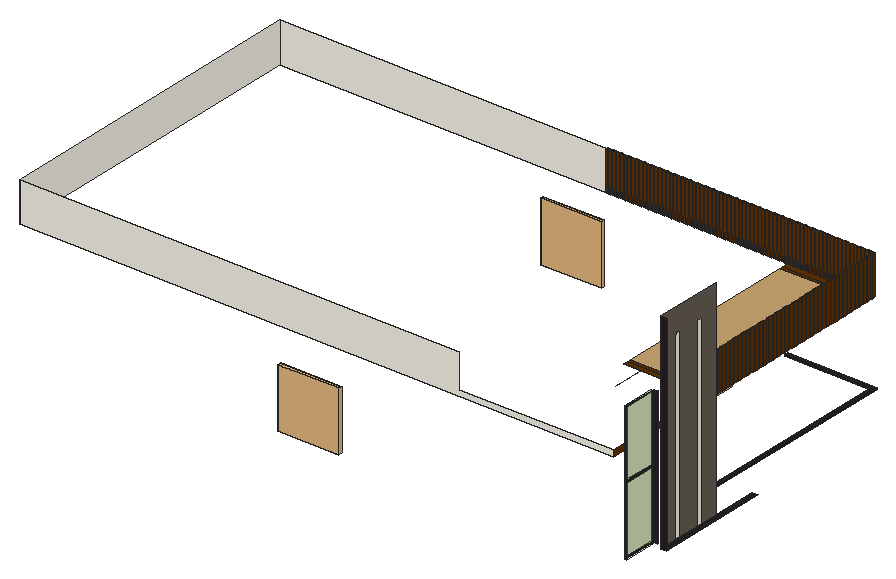
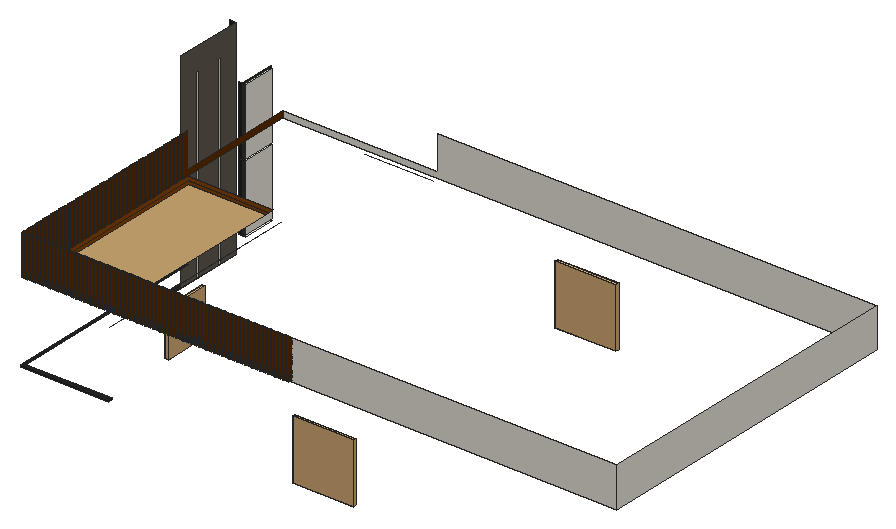
# SketchUp Ruby script. Lengths in inches.
U = 1.inch
M = Sketchup.active_model
def pt(a) = Geom::Point3d.new(a.map { |v| v * U })
def face(e, loops, mat)
  f = e.add_face(loops[0].map { |a| pt(a) })
  loops[1..].each { |l| e.add_face(l.map { |a| pt(a) }).erase! }
  f.material = f.back_material = mat if mat
  f
end
# faces: each face lists its corners as indices into pts; further lists are holes
def faces(e, pts, list, mat = nil) = list.each { |f| face(e, (f[0].is_a?(Array) ? f : [f]).map { |l| l.map { |i| pts[i] } }, mat) }
# xy, xz, yz: faces in a plane at the given z, y or x. An outline is a flat list of corners, or four numbers for a rectangle; further outlines are holes
def ring(l) = l.size == 4 ? [[l[0], l[1]], [l[2], l[1]], [l[2], l[3]], [l[0], l[3]]] : l.each_slice(2).to_a
def flat(e, list, mat, &to3) = list.each { |f| face(e, (f[0].is_a?(Array) ? f : [f]).map { |l| ring(l).map { |u, v| to3.(u, v) } }, mat) }
def xy(e, z, list, mat = nil) = flat(e, list, mat) { |x, y| [x, y, z] }
def xz(e, y, list, mat = nil) = flat(e, list, mat) { |x, z| [x, y, z] }
def yz(e, x, list, mat = nil) = flat(e, list, mat) { |y, z| [x, y, z] }
def lines(e, pts, list) = list.each { |a, b| e.add_line(pt(pts[a]), pt(pts[b])) }
# prism: a flat outline (further loops are holes) pulled along v
def prism(e, loops, v, mat = nil)
  f = face(e, loops, mat); d = Geom::Vector3d.new(v.map { |x| x * U })
  f.pushpull(f.normal.samedirection?(d) ? d.length : -d.length)
end
def box(e, o, s, mat = nil) = prism(e, [[o, [o[0] + s[0], o[1], o[2]], [o[0] + s[0], o[1] + s[1], o[2]], [o[0], o[1] + s[1], o[2]]]], [0, 0, s[2]], mat)
def at(x, y, z, deg = 0) = Geom::Transformation.translation(pt([x, y, z])) * Geom::Transformation.rotation(ORIGIN, Z_AXIS, deg.degrees)
def axes(o, x, y, z) = Geom::Transformation.new([*x, 0, *y, 0, *z, 0, *pt(o).to_a, 1])
def part(name) = M.definitions.add(name)
# library, detail: a bought-in or finely detailed component or shape, given as its bounding box
def library(name, o, s) = part(name).tap { |d| box(d.entities, o, s) }
def detail(e, o, s) = box(e.add_group.entities, o, s)
def put(e, d, t, mat = nil) = e.add_instance(d, t).tap { |i| i.material = mat if mat }
def group(e, t, mat = nil) = e.add_group.tap { |g| g.transformation = t; g.material = mat if mat }.entities
root = M.entities
M.materials.add("C01_Vanilla_Cream").color = [255, 251, 241]
M.materials.add("C08_Toffee_Ember").color = [102, 51, 0]
M.materials.add("Glass_Basic_01").color = [119, 186, 61]
M.materials["Glass_Basic_01"].alpha = 0.25
M.materials.add("Marble_07_1K").color = [36, 34, 36]
M.materials.add("Plaster_04_1K").color = [106, 98, 87]
M.materials.add("Plywood_08_1K").color = [202, 166, 113]
c1 = library("mesh-163",[-551.08,-704.17,-20.03],[1929.24,1401.85,86.96])
c2 = part("Group11")
put(c2.entities,c1,at(0,0,0))
xy(root,396,[[700,72,706,192]],"Marble_07_1K")
xy(root,407,[[700,25,702,59]],"C01_Vanilla_Cream")
xy(root,409,[[700,25,702,59]],"C01_Vanilla_Cream")
xy(root,420,[[693.41,144,696.41,144,696.41,360,603,360,603,357,693.41,357]],"Marble_07_1K")
xy(root,479,[[700,25,702,59]],"C01_Vanilla_Cream")
xy(root,481,[[700,25,702,59]],"C01_Vanilla_Cream")
xy(root,504,[[603,144,603,150,687.41,150,687.41,354,603,354,603,361.13,604.65,361.13,604.65,360,606.67,360,606.67,361.13,608.6875,361.13,608.6875,360,610.71,360,610.71,361.13,612.72,361.13,612.72,360,614.74,360,614.74,361.13,616.76,361.13,616.76,360,618.78,360,618.78,361.13,620.79,361.13,620.79,360,622.81,360,622.81,361.13,624.83,361.13,624.83,360,626.84,360,626.84,361.13,628.86,361.13,628.86,360,630.88,360,630.88,361.13,632.9,361.13,632.9,360,634.91,360,634.91,361.13,636.93,361.13,636.93,360,638.95,360,638.95,361.13,640.97,361.13,640.97,360,642.98,360,642.98,361,645,361,645,360,647.02,360,647.02,361,649.03,361,649.03,360,651.05,360,651.05,361,653.07,361,653.07,360,655.09,360,655.09,361,657.1,361,657.1,360,659.12,360,659.12,361,661.14,361,661.14,360,663.15,360,663.15,361,665.17,361,665.17,360,667.1875,360,667.1875,361,669.21,361,669.21,360,671.22,360,671.22,361,673.24,361,673.24,360,675.26,360,675.26,361,677.28,361,677.28,360,679.29,360,679.29,361,681.31,361,681.31,360,683.33,360,683.33,361,685.34,361,685.34,360,687.36,360,687.36,361,689.38,361,689.38,360,691.4,360,691.4,361,694.41,361,694.41,357.3,693.41,357.3,693.41,354.6,694.41,354.6,694.41,351.9,693.41,351.9,693.41,349.2,694.41,349.2,694.41,346.5,693.41,346.5,693.41,343.8,694.41,343.8,694.41,341.1,693.41,341.1,693.41,338.4,694.41,338.4,694.41,335.7,693.41,335.7,693.41,333,694.41,333,694.41,330.3,693.41,330.3,693.41,327.6,694.41,327.6,694.41,324.9,693.41,324.9,693.41,322.2,694.41,322.2,694.41,319.5,693.41,319.5,693.41,316.8,694.41,316.8,694.41,314.1,693.41,314.1,693.41,311.4,694.41,311.4,694.41,308.7,693.41,308.7,693.41,306,694.41,306,694.41,303.3,693.41,303.3,693.41,300.6,694.41,300.6,694.41,297.9,693.41,297.9,693.41,295.2,694.41,295.2,694.41,292.5,693.41,292.5,693.41,289.8,694.41,289.8,694.41,287.1,693.41,287.1,693.41,284.4,694.41,284.4,694.41,281.7,693.41,281.7,693.41,279,694.41,279,694.41,276.3,693.41,276.3,693.41,273.6,694.41,273.6,694.41,270.9,693.41,270.9,693.41,268.2,694.41,268.2,694.41,265.5,693.41,265.5,693.41,262.8,694.41,262.8,694.41,260.1,693.41,260.1,693.41,257.4,694.41,257.4,694.41,254.7,693.41,254.7,693.41,252,694.41,252,694.41,249.3,693.41,249.3,693.41,246.6,694.41,246.6,694.41,243.9,693.41,243.9,693.41,241.2,694.41,241.2,694.41,238.5,693.41,238.5,693.41,235.8,694.41,235.8,694.41,233.1,693.41,233.1,693.41,230.4,694.41,230.4,694.41,227.7,693.41,227.7,693.41,225,694.41,225,694.41,222.3,693.41,222.3,693.41,219.6,694.41,219.6,694.41,214.2,693.41,214.2,693.41,211.5,694.41,211.5,694.41,208.8,693.41,208.8,693.41,206.1,694.41,206.1,694.41,203.4,693.41,203.4,693.41,200.7,694.41,200.7,694.41,198,693.41,198,693.41,195.3,694.41,195.3,694.41,192.6,693.41,192.6,693.41,189.9,694.41,189.9,694.41,187.2,693.41,187.2,693.41,184.5,694.41,184.5,694.41,181.8,693.41,181.8,693.41,179.1,694.41,179.1,694.41,176.4,693.41,176.4,693.41,173.7,694.41,173.7,694.41,171,693.41,171,693.41,168.3,694.41,168.3,694.41,165.6,693.41,165.6,693.41,162.9,694.41,162.9,694.41,160.2,693.41,160.2,693.41,157.5,694.41,157.5,694.41,154.8,693.41,154.8,693.41,152.1,694.41,152.1,694.41,149.4,693.41,149.4,693.41,146.7,694.41,146.7,694.41,144],[603,150,603,154,683.41,154,683.41,350,603,350,603,354,687.41,354,687.41,150]],"C08_Toffee_Ember")
xy(root,504,[[603,154,683.41,350]],"Plywood_08_1K")
xz(root,18,[[69,504,693.41,504,693.41,510,531,510,531,546,69,546]],"C01_Vanilla_Cream")
xz(root,25,[[700,409,702,479],[700,481,702,551]],"C01_Vanilla_Cream")
xz(root,59,[[700,409,702,479],[700,481,702,551]],"C01_Vanilla_Cream")
xz(root,60,[[702,408,706,480],[702,480,706,552]],"Marble_07_1K")
xz(root,72,[[700,396,706,615]],"Marble_07_1K")
xz(root,144,[[693.41,504,694.41,510]],"C08_Toffee_Ember")
xz(root,146.7,[[693.41,504,694.41,510]],"C08_Toffee_Ember")
xz(root,149.4,[[693.41,504,694.41,510]],"C08_Toffee_Ember")
xz(root,152.1,[[693.41,504,694.41,510]],"C08_Toffee_Ember")
xz(root,154.8,[[693.41,504,694.41,510]],"C08_Toffee_Ember")
xz(root,157.5,[[693.41,504,694.41,510]],"C08_Toffee_Ember")
xz(root,160.2,[[693.41,504,694.41,510]],"C08_Toffee_Ember")
xz(root,162.9,[[693.41,504,694.41,510]],"C08_Toffee_Ember")
xz(root,165.6,[[693.41,504,694.41,510]],"C08_Toffee_Ember")
xz(root,168.3,[[693.41,504,694.41,510]],"C08_Toffee_Ember")
xz(root,171,[[693.41,504,694.41,510]],"C08_Toffee_Ember")
xz(root,173.7,[[693.41,504,694.41,510]],"C08_Toffee_Ember")
xz(root,176.4,[[693.41,504,694.41,510]],"C08_Toffee_Ember")
xz(root,179.1,[[693.41,504,694.41,510]],"C08_Toffee_Ember")
xz(root,181.8,[[693.41,504,694.41,510]],"C08_Toffee_Ember")
xz(root,184.5,[[693.41,504,694.41,510]],"C08_Toffee_Ember")
xz(root,187.2,[[693.41,504,694.41,510]],"C08_Toffee_Ember")
xz(root,189.9,[[693.41,504,694.41,510]],"C08_Toffee_Ember")
xz(root,192.6,[[693.41,504,694.41,510]],"C08_Toffee_Ember")
xz(root,195.3,[[693.41,504,694.41,510]],"C08_Toffee_Ember")
xz(root,198,[[693.41,504,694.41,510]],"C08_Toffee_Ember")
xz(root,200.7,[[693.41,504,694.41,510]],"C08_Toffee_Ember")
xz(root,203.4,[[693.41,504,694.41,510]],"C08_Toffee_Ember")
xz(root,206.1,[[693.41,504,694.41,510]],"C08_Toffee_Ember")
xz(root,208.8,[[693.41,504,694.41,510]],"C08_Toffee_Ember")
xz(root,211.5,[[693.41,504,694.41,510]],"C08_Toffee_Ember")
xz(root,214.2,[[693.41,504,694.41,510]],"C08_Toffee_Ember")
xz(root,219.6,[[693.41,504,694.41,510]],"C08_Toffee_Ember")
xz(root,222.3,[[693.41,504,694.41,510]],"C08_Toffee_Ember")
xz(root,225,[[693.41,504,694.41,510]],"C08_Toffee_Ember")
xz(root,227.7,[[693.41,504,694.41,510]],"C08_Toffee_Ember")
xz(root,230.4,[[693.41,504,694.41,510]],"C08_Toffee_Ember")
xz(root,233.1,[[693.41,504,694.41,510]],"C08_Toffee_Ember")
xz(root,235.8,[[693.41,504,694.41,510]],"C08_Toffee_Ember")
xz(root,238.5,[[693.41,504,694.41,510]],"C08_Toffee_Ember")
xz(root,241.2,[[693.41,504,694.41,510]],"C08_Toffee_Ember")
xz(root,243.9,[[693.41,504,694.41,510]],"C08_Toffee_Ember")
xz(root,246.6,[[693.41,504,694.41,510]],"C08_Toffee_Ember")
xz(root,249.3,[[693.41,504,694.41,510]],"C08_Toffee_Ember")
xz(root,252,[[693.41,504,694.41,510]],"C08_Toffee_Ember")
xz(root,254.7,[[693.41,504,694.41,510]],"C08_Toffee_Ember")
xz(root,257.4,[[693.41,504,694.41,510]],"C08_Toffee_Ember")
xz(root,260.1,[[693.41,504,694.41,510]],"C08_Toffee_Ember")
xz(root,262.8,[[693.41,504,694.41,510]],"C08_Toffee_Ember")
xz(root,265.5,[[693.41,504,694.41,510]],"C08_Toffee_Ember")
xz(root,268.2,[[693.41,504,694.41,510]],"C08_Toffee_Ember")
xz(root,270.9,[[693.41,504,694.41,510]],"C08_Toffee_Ember")
xz(root,273.6,[[693.41,504,694.41,510]],"C08_Toffee_Ember")
xz(root,276.3,[[693.41,504,694.41,510]],"C08_Toffee_Ember")
xz(root,279,[[693.41,504,694.41,510]],"C08_Toffee_Ember")
xz(root,281.7,[[693.41,504,694.41,510]],"C08_Toffee_Ember")
xz(root,284.4,[[693.41,504,694.41,510]],"C08_Toffee_Ember")
xz(root,287.1,[[693.41,504,694.41,510]],"C08_Toffee_Ember")
xz(root,289.8,[[693.41,504,694.41,510]],"C08_Toffee_Ember")
xz(root,292.5,[[693.41,504,694.41,510]],"C08_Toffee_Ember")
xz(root,295.2,[[693.41,504,694.41,510]],"C08_Toffee_Ember")
xz(root,297.9,[[693.41,504,694.41,510]],"C08_Toffee_Ember")
xz(root,300.6,[[693.41,504,694.41,510]],"C08_Toffee_Ember")
xz(root,303.3,[[693.41,504,694.41,510]],"C08_Toffee_Ember")
xz(root,306,[[693.41,504,694.41,510]],"C08_Toffee_Ember")
xz(root,308.7,[[693.41,504,694.41,510]],"C08_Toffee_Ember")
xz(root,311.4,[[693.41,504,694.41,510]],"C08_Toffee_Ember")
xz(root,314.1,[[693.41,504,694.41,510]],"C08_Toffee_Ember")
xz(root,316.8,[[693.41,504,694.41,510]],"C08_Toffee_Ember")
xz(root,319.5,[[693.41,504,694.41,510]],"C08_Toffee_Ember")
xz(root,322.2,[[693.41,504,694.41,510]],"C08_Toffee_Ember")
xz(root,324.9,[[693.41,504,694.41,510]],"C08_Toffee_Ember")
xz(root,327.6,[[693.41,504,694.41,510]],"C08_Toffee_Ember")
xz(root,330.3,[[693.41,504,694.41,510]],"C08_Toffee_Ember")
xz(root,333,[[693.41,504,694.41,510]],"C08_Toffee_Ember")
xz(root,335.7,[[693.41,504,694.41,510]],"C08_Toffee_Ember")
xz(root,338.4,[[693.41,504,694.41,510]],"C08_Toffee_Ember")
xz(root,341.1,[[693.41,504,694.41,510]],"C08_Toffee_Ember")
xz(root,343.8,[[693.41,504,694.41,510]],"C08_Toffee_Ember")
xz(root,346.5,[[693.41,504,694.41,510]],"C08_Toffee_Ember")
xz(root,349.2,[[693.41,504,694.41,510]],"C08_Toffee_Ember")
xz(root,351.9,[[693.41,504,694.41,510]],"C08_Toffee_Ember")
xz(root,354.6,[[693.41,504,694.41,510]],"C08_Toffee_Ember")
xz(root,357,[[603,418,693.41,420]],"Marble_07_1K")
xz(root,357.3,[[693.41,504,694.41,510]],"C08_Toffee_Ember")
xz(root,360,[[69,504,411,546]],"C01_Vanilla_Cream")
xz(root,360,[[411,504,413.02,546],[415.03,504,417.05,546],[419.07,504,421.09,546],[423.1,504,425.12,546],[427.14,504,429.16,546],
  [431.17,504,433.19,546],[435.21,504,437.22,546],[439.24,504,441.26,546],[443.28,504,445.29,546],[447.31,504,449.33,546],
  [451.34,504,453.36,546],[455.38,504,457.4,546],[459.41,504,461.43,546],[463.45,504,465.47,546],[467.48,504,469.5,546],
  [471.52,504,473.53,546],[475.55,504,477.57,546],[479.59,504,481.6,546],[483.62,504,485.64,546],[487.66,504,489.67,546],
  [491.69,504,493.71,546],[495.72,504,497.74,546],[499.76,504,501.78,546],[503.79,504,505.81,546],[507.83,504,509.84,546],
  [511.86,504,513.88,546],[515.9,504,517.91,546],[519.93,504,521.95,546],[523.97,504,525.98,546],[528,504,530.02,546],
  [532.03,504,534.05,546],[536.07,504,538.09,546],[540.1,504,542.12,546],[544.14,504,546.15,546],[548.17,504,550.1875,546],
  [552.21,504,554.22,546],[556.24,504,558.26,546],[560.28,504,562.29,546],[564.31,504,566.33,546],[568.34,504,570.36,546],
  [572.38,504,574.4,546],[576.41,504,578.43,546],[580.45,504,582.47,546],[584.48,504,586.5,546],[588.52,504,590.53,546],
  [592.55,504,594.57,546],[596.59,504,598.6,546],[600.62,504,602.64,546],[604.65,504,606.67,546],[608.6875,504,610.71,546],
  [612.72,504,614.74,546],[616.76,504,618.78,546],[620.79,504,622.81,546],[624.83,504,626.84,546],[628.86,504,630.88,546],
  [632.9,504,634.91,546],[636.93,504,638.95,546],[640.97,504,642.98,546],[645,504,647.02,546],[649.03,504,651.05,546],
  [653.07,504,655.09,546],[657.1,504,659.12,546],[661.14,504,663.15,546],[665.17,504,667.1875,546],[669.21,504,671.22,546],
  [673.24,504,675.26,546],[677.28,504,679.29,546],[681.31,504,683.33,546],[685.34,504,687.36,546],[689.38,504,691.4,546]],"C08_Toffee_Ember")
xz(root,360,[[603,418,696.41,420]],"Marble_07_1K")
xz(root,361,[[642.98,504,645,546],[647.02,504,649.03,546],[651.05,504,653.07,546],[655.09,504,657.1,546],[659.12,504,661.14,546],
  [663.15,504,665.17,546],[667.1875,504,669.21,546],[671.22,504,673.24,546],[675.26,504,677.28,546],[679.29,504,681.31,546],
  [683.33,504,685.34,546],[687.36,504,689.38,546],[691.4,504,694.41,546]],"C08_Toffee_Ember")
xz(root,361.09,[[429.16,504,431.17,546],[433.19,504,435.21,546],[437.22,504,439.24,546],[441.26,504,443.28,546],[445.29,504,447.31,546],
  [449.33,504,451.34,546],[453.36,504,455.38,546],[457.4,504,459.41,546],[461.43,504,463.45,546],[465.47,504,467.48,546],
  [469.5,504,471.52,546]],"C08_Toffee_Ember")
xz(root,361.11,[[413.02,504,415.03,546],[417.05,504,419.07,546],[421.09,504,423.1,546],[425.12,504,427.14,546]],"C08_Toffee_Ember")
xz(root,361.13,[[598.6,504,600.62,546],[602.64,504,604.65,546],[606.67,504,608.6875,546],[610.71,504,612.72,546],[614.74,504,616.76,546],
  [618.78,504,620.79,546],[622.81,504,624.83,546],[626.84,504,628.86,546],[630.88,504,632.9,546],[634.91,504,636.93,546],
  [638.95,504,640.97,546]],"C08_Toffee_Ember")
xz(root,361.1875,[[473.53,504,475.55,546],[477.57,504,479.59,546],[481.6,504,483.62,546],[485.64,504,487.66,546],[489.67,504,491.69,546],
  [493.71,504,495.72,546],[497.74,504,499.76,546],[501.78,504,503.79,546],[505.81,504,507.83,546],[509.84,504,511.86,546],
  [513.88,504,515.9,546],[517.91,504,519.93,546],[521.95,504,523.97,546],[525.98,504,528,546],[530.02,504,532.03,546],
  [534.05,504,536.07,546],[538.09,504,540.1,546],[542.12,504,544.14,546],[546.15,504,548.17,546],[550.1875,504,552.21,546],
  [554.22,504,556.24,546],[558.26,504,560.28,546],[562.29,504,564.31,546],[566.33,504,568.34,546],[570.36,504,572.38,546],
  [574.4,504,576.41,546],[578.43,504,580.45,546],[582.47,504,584.48,546],[586.5,504,588.52,546],[590.53,504,592.55,546],
  [594.57,504,596.59,546]],"C08_Toffee_Ember")
yz(root,69,[[18,504,360,546]],"C01_Vanilla_Cream")
yz(root,413.02,[[360,504,361.11,510]],"C08_Toffee_Ember")
yz(root,415.03,[[360,504,361.11,510]],"C08_Toffee_Ember")
yz(root,417.05,[[360,504,361.11,510]],"C08_Toffee_Ember")
yz(root,419.07,[[360,504,361.11,510]],"C08_Toffee_Ember")
yz(root,421.09,[[360,504,361.11,510]],"C08_Toffee_Ember")
yz(root,423.1,[[360,504,361.11,510]],"C08_Toffee_Ember")
yz(root,425.12,[[360,504,361.11,510]],"C08_Toffee_Ember")
yz(root,427.14,[[360,504,361.11,510]],"C08_Toffee_Ember")
yz(root,429.16,[[360,504,361.09,510]],"C08_Toffee_Ember")
yz(root,431.17,[[360,504,361.09,510]],"C08_Toffee_Ember")
yz(root,433.19,[[360,504,361.09,510]],"C08_Toffee_Ember")
yz(root,435.21,[[360,504,361.09,510]],"C08_Toffee_Ember")
yz(root,437.22,[[360,504,361.09,510]],"C08_Toffee_Ember")
yz(root,439.24,[[360,504,361.09,510]],"C08_Toffee_Ember")
yz(root,441.26,[[360,504,361.09,510]],"C08_Toffee_Ember")
yz(root,443.28,[[360,504,361.09,510]],"C08_Toffee_Ember")
yz(root,445.29,[[360,504,361.09,510]],"C08_Toffee_Ember")
yz(root,447.31,[[360,504,361.09,510]],"C08_Toffee_Ember")
yz(root,449.33,[[360,504,361.09,510]],"C08_Toffee_Ember")
yz(root,451.34,[[360,504,361.09,510]],"C08_Toffee_Ember")
yz(root,453.36,[[360,504,361.09,510]],"C08_Toffee_Ember")
yz(root,455.38,[[360,504,361.09,510]],"C08_Toffee_Ember")
yz(root,457.4,[[360,504,361.09,510]],"C08_Toffee_Ember")
yz(root,459.41,[[360,504,361.09,510]],"C08_Toffee_Ember")
yz(root,461.43,[[360,504,361.09,510]],"C08_Toffee_Ember")
yz(root,463.45,[[360,504,361.09,510]],"C08_Toffee_Ember")
yz(root,465.47,[[360,504,361.09,510]],"C08_Toffee_Ember")
yz(root,467.48,[[360,504,361.09,510]],"C08_Toffee_Ember")
yz(root,469.5,[[360,504,361.09,510]],"C08_Toffee_Ember")
yz(root,471.52,[[360,504,361.09,510]],"C08_Toffee_Ember")
yz(root,473.53,[[360,504,361.1875,510]],"C08_Toffee_Ember")
yz(root,475.55,[[360,504,361.1875,510]],"C08_Toffee_Ember")
yz(root,477.57,[[360,504,361.1875,510]],"C08_Toffee_Ember")
yz(root,479.59,[[360,504,361.1875,510]],"C08_Toffee_Ember")
yz(root,481.6,[[360,504,361.1875,510]],"C08_Toffee_Ember")
yz(root,483.62,[[360,504,361.1875,510]],"C08_Toffee_Ember")
yz(root,485.64,[[360,504,361.1875,510]],"C08_Toffee_Ember")
yz(root,487.66,[[360,504,361.1875,510]],"C08_Toffee_Ember")
yz(root,489.67,[[360,504,361.1875,510]],"C08_Toffee_Ember")
yz(root,491.69,[[360,504,361.1875,510]],"C08_Toffee_Ember")
yz(root,493.71,[[360,504,361.1875,510]],"C08_Toffee_Ember")
yz(root,495.72,[[360,504,361.1875,510]],"C08_Toffee_Ember")
yz(root,497.74,[[360,504,361.1875,510]],"C08_Toffee_Ember")
yz(root,499.76,[[360,504,361.1875,510]],"C08_Toffee_Ember")
yz(root,501.78,[[360,504,361.1875,510]],"C08_Toffee_Ember")
yz(root,503.79,[[360,504,361.1875,510]],"C08_Toffee_Ember")
yz(root,505.81,[[360,504,361.1875,510]],"C08_Toffee_Ember")
yz(root,507.83,[[360,504,361.1875,510]],"C08_Toffee_Ember")
yz(root,509.84,[[360,504,361.1875,510]],"C08_Toffee_Ember")
yz(root,511.86,[[360,504,361.1875,510]],"C08_Toffee_Ember")
yz(root,513.88,[[360,504,361.1875,510]],"C08_Toffee_Ember")
yz(root,515.9,[[360,504,361.1875,510]],"C08_Toffee_Ember")
yz(root,517.91,[[360,504,361.1875,510]],"C08_Toffee_Ember")
yz(root,519.93,[[360,504,361.1875,510]],"C08_Toffee_Ember")
yz(root,521.95,[[360,504,361.1875,510]],"C08_Toffee_Ember")
yz(root,523.97,[[360,504,361.1875,510]],"C08_Toffee_Ember")
yz(root,525.98,[[360,504,361.1875,510]],"C08_Toffee_Ember")
yz(root,528,[[360,504,361.1875,510]],"C08_Toffee_Ember")
yz(root,530.02,[[360,504,361.1875,510]],"C08_Toffee_Ember")
yz(root,532.03,[[360,504,361.1875,510]],"C08_Toffee_Ember")
yz(root,534.05,[[360,504,361.1875,510]],"C08_Toffee_Ember")
yz(root,536.07,[[360,504,361.1875,510]],"C08_Toffee_Ember")
yz(root,538.09,[[360,504,361.1875,510]],"C08_Toffee_Ember")
yz(root,540.1,[[360,504,361.1875,510]],"C08_Toffee_Ember")
yz(root,542.12,[[360,504,361.1875,510]],"C08_Toffee_Ember")
yz(root,544.14,[[360,504,361.1875,510]],"C08_Toffee_Ember")
yz(root,546.15,[[360,504,361.1875,510]],"C08_Toffee_Ember")
yz(root,548.17,[[360,504,361.1875,510]],"C08_Toffee_Ember")
yz(root,550.1875,[[360,504,361.1875,510]],"C08_Toffee_Ember")
yz(root,552.21,[[360,504,361.1875,510]],"C08_Toffee_Ember")
yz(root,554.22,[[360,504,361.1875,510]],"C08_Toffee_Ember")
yz(root,556.24,[[360,504,361.1875,510]],"C08_Toffee_Ember")
yz(root,558.26,[[360,504,361.1875,510]],"C08_Toffee_Ember")
yz(root,560.28,[[360,504,361.1875,510]],"C08_Toffee_Ember")
yz(root,562.29,[[360,504,361.1875,510]],"C08_Toffee_Ember")
yz(root,564.31,[[360,504,361.1875,510]],"C08_Toffee_Ember")
yz(root,566.33,[[360,504,361.1875,510]],"C08_Toffee_Ember")
yz(root,568.34,[[360,504,361.1875,510]],"C08_Toffee_Ember")
yz(root,570.36,[[360,504,361.1875,510]],"C08_Toffee_Ember")
yz(root,572.38,[[360,504,361.1875,510]],"C08_Toffee_Ember")
yz(root,574.4,[[360,504,361.1875,510]],"C08_Toffee_Ember")
yz(root,576.41,[[360,504,361.1875,510]],"C08_Toffee_Ember")
yz(root,578.43,[[360,504,361.1875,510]],"C08_Toffee_Ember")
yz(root,580.45,[[360,504,361.1875,510]],"C08_Toffee_Ember")
yz(root,582.47,[[360,504,361.1875,510]],"C08_Toffee_Ember")
yz(root,584.48,[[360,504,361.1875,510]],"C08_Toffee_Ember")
yz(root,586.5,[[360,504,361.1875,510]],"C08_Toffee_Ember")
yz(root,588.52,[[360,504,361.1875,510]],"C08_Toffee_Ember")
yz(root,590.53,[[360,504,361.1875,510]],"C08_Toffee_Ember")
yz(root,592.55,[[360,504,361.1875,510]],"C08_Toffee_Ember")
yz(root,594.57,[[360,504,361.1875,510]],"C08_Toffee_Ember")
yz(root,596.59,[[360,504,361.1875,510]],"C08_Toffee_Ember")
yz(root,598.6,[[360,504,361.13,510]],"C08_Toffee_Ember")
yz(root,600.62,[[360,504,361.13,510]],"C08_Toffee_Ember")
yz(root,602.64,[[360,504,361.13,510]],"C08_Toffee_Ember")
yz(root,603,[[357,418,360,420]],"Marble_07_1K")
yz(root,604.65,[[360,504,361.13,510]],"C08_Toffee_Ember")
yz(root,606.67,[[360,504,361.13,510]],"C08_Toffee_Ember")
yz(root,608.6875,[[360,504,361.13,510]],"C08_Toffee_Ember")
yz(root,610.71,[[360,504,361.13,510]],"C08_Toffee_Ember")
yz(root,612.72,[[360,504,361.13,510]],"C08_Toffee_Ember")
yz(root,614.74,[[360,504,361.13,510]],"C08_Toffee_Ember")
yz(root,616.76,[[360,504,361.13,510]],"C08_Toffee_Ember")
yz(root,618.78,[[360,504,361.13,510]],"C08_Toffee_Ember")
yz(root,620.79,[[360,504,361.13,510]],"C08_Toffee_Ember")
yz(root,622.81,[[360,504,361.13,510]],"C08_Toffee_Ember")
yz(root,624.83,[[360,504,361.13,510]],"C08_Toffee_Ember")
yz(root,626.84,[[360,504,361.13,510]],"C08_Toffee_Ember")
yz(root,628.86,[[360,504,361.13,510]],"C08_Toffee_Ember")
yz(root,630.88,[[360,504,361.13,510]],"C08_Toffee_Ember")
yz(root,632.9,[[360,504,361.13,510]],"C08_Toffee_Ember")
yz(root,634.91,[[360,504,361.13,510]],"C08_Toffee_Ember")
yz(root,636.93,[[360,504,361.13,510]],"C08_Toffee_Ember")
yz(root,638.95,[[360,504,361.13,510]],"C08_Toffee_Ember")
yz(root,640.97,[[360,504,361.13,510]],"C08_Toffee_Ember")
yz(root,642.98,[[360,504,361,510]],"C08_Toffee_Ember")
yz(root,645,[[360,504,361,510]],"C08_Toffee_Ember")
yz(root,647.02,[[360,504,361,510]],"C08_Toffee_Ember")
yz(root,649.03,[[360,504,361,510]],"C08_Toffee_Ember")
yz(root,651.05,[[360,504,361,510]],"C08_Toffee_Ember")
yz(root,653.07,[[360,504,361,510]],"C08_Toffee_Ember")
yz(root,655.09,[[360,504,361,510]],"C08_Toffee_Ember")
yz(root,657.1,[[360,504,361,510]],"C08_Toffee_Ember")
yz(root,659.12,[[360,504,361,510]],"C08_Toffee_Ember")
yz(root,661.14,[[360,504,361,510]],"C08_Toffee_Ember")
yz(root,663.15,[[360,504,361,510]],"C08_Toffee_Ember")
yz(root,665.17,[[360,504,361,510]],"C08_Toffee_Ember")
yz(root,667.1875,[[360,504,361,510]],"C08_Toffee_Ember")
yz(root,669.21,[[360,504,361,510]],"C08_Toffee_Ember")
yz(root,671.22,[[360,504,361,510]],"C08_Toffee_Ember")
yz(root,673.24,[[360,504,361,510]],"C08_Toffee_Ember")
yz(root,675.26,[[360,504,361,510]],"C08_Toffee_Ember")
yz(root,677.28,[[360,504,361,510]],"C08_Toffee_Ember")
yz(root,679.29,[[360,504,361,510]],"C08_Toffee_Ember")
yz(root,681.31,[[360,504,361,510]],"C08_Toffee_Ember")
yz(root,683.33,[[360,504,361,510]],"C08_Toffee_Ember")
yz(root,685.34,[[360,504,361,510]],"C08_Toffee_Ember")
yz(root,687.36,[[360,504,361,510]],"C08_Toffee_Ember")
yz(root,689.38,[[360,504,361,510]],"C08_Toffee_Ember")
yz(root,691.4,[[360,504,361,510]],"C08_Toffee_Ember")
yz(root,693.41,[[18,504,144,510],[146.7,504,149.4,546],[152.1,504,154.8,546],[157.5,504,160.2,546],[162.9,504,165.6,546],
  [168.3,504,171,546],[173.7,504,176.4,546],[179.1,504,181.8,546],[184.5,504,187.2,546],[189.9,504,192.6,546],
  [195.3,504,198,546],[200.7,504,203.4,546],[206.1,504,208.8,546],[211.5,504,214.2,546],[219.6,504,222.3,546],
  [225,504,227.7,546],[230.4,504,233.1,546],[235.8,504,238.5,546],[241.2,504,243.9,546],[246.6,504,249.3,546],
  [252,504,254.7,546],[257.4,504,260.1,546],[262.8,504,265.5,546],[268.2,504,270.9,546],[273.6,504,276.3,546],
  [279,504,281.7,546],[284.4,504,287.1,546],[289.8,504,292.5,546],[295.2,504,297.9,546],[300.6,504,303.3,546],
  [306,504,308.7,546],[311.4,504,314.1,546],[316.8,504,319.5,546],[322.2,504,324.9,546],[327.6,504,330.3,546],
  [333,504,335.7,546],[338.4,504,341.1,546],[343.8,504,346.5,546],[349.2,504,351.9,546],[354.6,504,357.3,546]],"C08_Toffee_Ember")
yz(root,694.41,[[144,504,146.7,546],[149.4,504,152.1,546],[154.8,504,157.5,546],[160.2,504,162.9,546],[165.6,504,168.3,546],
  [171,504,173.7,546],[176.4,504,179.1,546],[181.8,504,184.5,546],[187.2,504,189.9,546],[192.6,504,195.3,546],
  [198,504,200.7,546],[203.4,504,206.1,546],[208.8,504,211.5,546],[214.2,504,216.9,546],[216.9,504,219.6,546],
  [222.3,504,225,546],[227.7,504,230.4,546],[233.1,504,235.8,546],[238.5,504,241.2,546],[243.9,504,246.6,546],
  [249.3,504,252,546],[254.7,504,257.4,546],[260.1,504,262.8,546],[265.5,504,268.2,546],[270.9,504,273.6,546],
  [276.3,504,279,546],[281.7,504,284.4,546],[287.1,504,289.8,546],[292.5,504,295.2,546],[297.9,504,300.6,546],
  [303.3,504,306,546],[308.7,504,311.4,546],[314.1,504,316.8,546],[319.5,504,322.2,546],[324.9,504,327.6,546],
  [330.3,504,333,546],[335.7,504,338.4,546],[341.1,504,343.8,546],[346.5,504,349.2,546],[351.9,504,354.6,546],
  [357.3,504,361,546]],"C08_Toffee_Ember")
yz(root,696.41,[[144,418,360,420]],"Marble_07_1K")
yz(root,700,[[92,396,96,590.1],[120,396,124,590.1],[25,409,59,479],[25,481,59,551]],"C01_Vanilla_Cream")
yz(root,700,[[72,396,92,396,92,590.1,96,590.1,96,396,120,396,120,590.1,124,590.1,124,396,144,396,144,615,72,615]],"Plaster_04_1K")
yz(root,702,[[25,409,59,479],[25,481,59,551]],"Glass_Basic_01")
yz(root,702,[[[24,408,60,480],[25,409,59,479]],[[24,480,60,552],[25,481,59,551]]],"Marble_07_1K")
p = [[531,24,504],[603,24,504],[603,133.77,487.96],[603,360,487.96]]
lines(root,p,[[0,1],[2,3]])
put(root,c2,axes([388.72,15.37,438.18],[-0.03317,0,0],[0,0,0.04465],[0,0.03937,0]))
put(root,c2,axes([388.72,360.79,443.44],[-0.03317,0,0],[0,0,0.04465],[0,0.03937,0]))
put(root,c2,axes([603.79,247.71,447.59],[0,0.02488,0],[0,0,0.0342],[0.03937,0,0]))
